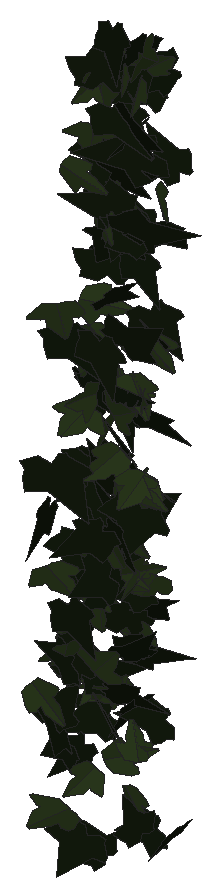
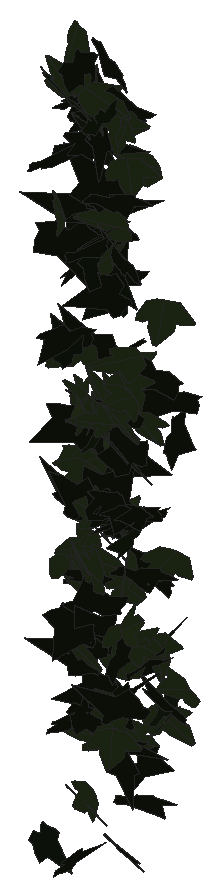
# SketchUp Ruby script. Lengths in inches.
U = 1.inch
M = Sketchup.active_model
def pt(a) = Geom::Point3d.new(a.map { |v| v * U })
def face(e, loops, mat)
  f = e.add_face(loops[0].map { |a| pt(a) })
  loops[1..].each { |l| e.add_face(l.map { |a| pt(a) }).erase! }
  f.material = f.back_material = mat if mat
  f
end
# faces: each face lists its corners as indices into pts; further lists are holes
def faces(e, pts, list, mat = nil) = list.each { |f| face(e, (f[0].is_a?(Array) ? f : [f]).map { |l| l.map { |i| pts[i] } }, mat) }
# xy, xz, yz: faces in a plane at the given z, y or x. An outline is a flat list of corners, or four numbers for a rectangle; further outlines are holes
def ring(l) = l.size == 4 ? [[l[0], l[1]], [l[2], l[1]], [l[2], l[3]], [l[0], l[3]]] : l.each_slice(2).to_a
def flat(e, list, mat, &to3) = list.each { |f| face(e, (f[0].is_a?(Array) ? f : [f]).map { |l| ring(l).map { |u, v| to3.(u, v) } }, mat) }
def xy(e, z, list, mat = nil) = flat(e, list, mat) { |x, y| [x, y, z] }
def xz(e, y, list, mat = nil) = flat(e, list, mat) { |x, z| [x, y, z] }
def yz(e, x, list, mat = nil) = flat(e, list, mat) { |y, z| [x, y, z] }
def lines(e, pts, list) = list.each { |a, b| e.add_line(pt(pts[a]), pt(pts[b])) }
# prism: a flat outline (further loops are holes) pulled along v
def prism(e, loops, v, mat = nil)
  f = face(e, loops, mat); d = Geom::Vector3d.new(v.map { |x| x * U })
  f.pushpull(f.normal.samedirection?(d) ? d.length : -d.length)
end
def box(e, o, s, mat = nil) = prism(e, [[o, [o[0] + s[0], o[1], o[2]], [o[0] + s[0], o[1] + s[1], o[2]], [o[0], o[1] + s[1], o[2]]]], [0, 0, s[2]], mat)
def at(x, y, z, deg = 0) = Geom::Transformation.translation(pt([x, y, z])) * Geom::Transformation.rotation(ORIGIN, Z_AXIS, deg.degrees)
def axes(o, x, y, z) = Geom::Transformation.new([*x, 0, *y, 0, *z, 0, *pt(o).to_a, 1])
def part(name) = M.definitions.add(name)
# library, detail: a bought-in or finely detailed component or shape, given as its bounding box
def library(name, o, s) = part(name).tap { |d| box(d.entities, o, s) }
def detail(e, o, s) = box(e.add_group.entities, o, s)
def put(e, d, t, mat = nil) = e.add_instance(d, t).tap { |i| i.material = mat if mat }
def group(e, t, mat = nil) = e.add_group.tap { |g| g.transformation = t; g.material = mat if mat }.entities
root = M.entities
M.materials.add("1026 AP 7946 SUNNY SIDE UP").color = [254, 231, 186]
M.materials.add("efeu1").color = [18, 25, 13]
M.materials.add("efeu2").color = [43, 57, 29]
c1 = part("ivyleaf_10")
p = [[0,0.5,-0.03],[-0.0625,2.02,-0.43],[-0.19,2.01,-0.46],[-0.54,1.05,-0.29],[-0.52,0.625,-0.18],[-0.83,0.76,-0.28],
  [-1.16,0.64,-0.33],[-1.15,0.33,-0.24],[-0.77,-0.39,0.02],[-0.3,-0.51,0.16],[0.04,-0.48,0.23],[-0.02,2.01,-0.4375],
  [-0.06,2.01,-0.43],[0.04,-0.49,0.23],[0.67,-0.49,0.14],[1.38,0.36,-0.2],[1.375,0.51,-0.24],[0.81,0.65,-0.19],
  [0.62,0.59,-0.15],[0.6,1.09,-0.28],[0.5,1.23,-0.31]]
faces(c1.entities,p,[[0,1,2,3,4,5,6,7,8,9,10],[11,12,0,13,14,15,16,17,18,19,20]],"efeu2")
c2 = part("ivyleaf_9")
p = [[1.54,2.16,1.25],[1.36,2.04,1.19],[-0.21,0.99,0.68],[-0.71,1.11,0.82],[-0.85,0.86,0.67],[-0.8,0.17,0.21],
  [-0.9,-0.01,0.1],[-0.67,-0.16,-0.02],[-0.08,-0.08,-0.05],[-0.03,-0.6,-0.4],[0.65,-0.88,-0.66],[0.83,-0.6,-0.49],
  [1.29,-0.42,-0.43],[1.8125,-0.07,-0.26],[1.21,0.44,0.15]]
faces(c2.entities,p,[[0,1,2,3,4,5,6,7,8,9,10,11,12,13,14]],"efeu1")
put(root,c1,axes([117.14,209.02,253.63],[-0.27587,-0.09025,0.21248],[-0.2515,-0.13497,-0.20129],[0.25018,-0.23519,0.03195]),"1026 AP 7946 SUNNY SIDE UP")
put(root,c2,axes([116.72,209.19,259.3],[-0.09999,0.04613,-0.32791],[0.33476,-0.23752,-0.08061],[-0.37961,-0.22161,0.01529]),"1026 AP 7946 SUNNY SIDE UP")
put(root,c2,axes([116.73,209.31,260.1],[-0.08354,-0.22855,-0.23884],[0.13648,0.21511,-0.23903],[0.49187,-0.09851,0.02576]),"1026 AP 7946 SUNNY SIDE UP")
put(root,c2,axes([117.36,209.79,258.8125],[-0.01614,-0.03063,-0.29387],[0.02416,-0.28492,0.0293],[-0.4502,-0.01419,0.01211]),"1026 AP 7946 SUNNY SIDE UP")
put(root,c2,axes([116.63,209.875,257.04],[-0.13329,-0.07492,-0.27678],[0.42285,0.05093,-0.10191],[0.11393,-0.27667,0.0544]),"1026 AP 7946 SUNNY SIDE UP")
put(root,c2,axes([117.24,210.14,257.74],[-0.16853,-0.15358,0.22708],[-0.17197,-0.19285,-0.19357],[0.38707,-0.15254,0.01287]),"1026 AP 7946 SUNNY SIDE UP")
put(root,c2,axes([116.16,210.13,254.47],[-0.02015,-0.19103,0.2175],[0.01022,-0.21257,-0.19797],[0.44885,-0.00374,0.01427]),"1026 AP 7946 SUNNY SIDE UP")
put(root,c2,axes([116.83,210.07,252.57],[-0.34327,-0.1662,0.00271],[0.01829,-0.02116,-0.28171],[0.26076,-0.21731,0.02333]),"1026 AP 7946 SUNNY SIDE UP")
put(root,c1,axes([115.79,210.04,255.05],[0.24848,0.01045,0.24141],[0.3686,-0.01472,-0.16231],[0.01003,0.2822,-0.01575]),"1026 AP 7946 SUNNY SIDE UP")
put(root,c1,axes([116.86,210.15,253.78],[0.15228,0.13186,-0.22572],[-0.17084,-0.19175,-0.16891],[-0.36512,0.14472,-0.01511]),"1026 AP 7946 SUNNY SIDE UP")
put(root,c2,axes([116.27,210.23,254.125],[0.13204,-0.16753,-0.18657],[0.14401,-0.15539,0.19193],[-0.35903,-0.12394,0.00837]),"1026 AP 7946 SUNNY SIDE UP")
put(root,c1,axes([116.77,210.31,261.03],[-0.00319,-0.02129,-0.30481],[-0.14173,-0.28172,0.01989],[-0.44418,0.09004,-0.00415]),"1026 AP 7946 SUNNY SIDE UP")
put(root,c1,axes([116.09,210.06,257.49],[-0.28402,-0.16723,-0.15757],[0.21516,0.07393,-0.25088],[0.2828,-0.2242,0.03263]),"1026 AP 7946 SUNNY SIDE UP")
put(root,c2,axes([116.29,210.31,255.66],[0.07807,-0.27122,-0.04217],[0.04896,-0.03419,0.28275],[-0.42815,-0.05336,0.02465]),"1026 AP 7946 SUNNY SIDE UP")
put(root,c1,axes([116.8,210.42,258.17],[-0.04534,-0.03091,-0.3116],[-0.03095,-0.30283,0.03206],[-0.4768,0.0226,0.02755]),"1026 AP 7946 SUNNY SIDE UP")
put(root,c2,axes([116.07,210.14,254.59],[-0.25331,0.18158,0.13881],[0.15811,-0.08925,0.24913],[0.31737,0.18939,-0.01332]),"1026 AP 7946 SUNNY SIDE UP")
put(root,c1,axes([116.19,210.3125,255.9],[-0.12614,-0.28371,-0.00245],[0.01409,-0.00173,-0.30361],[0.44589,-0.08021,0.0089]),"1026 AP 7946 SUNNY SIDE UP")
put(root,c1,axes([116.03,210.33,262.46],[-0.31797,-0.22697,-0.0564],[0.08029,0.02594,-0.3123],[0.35776,-0.20755,0.01996]),"1026 AP 7946 SUNNY SIDE UP")
put(root,c2,axes([117.1875,210.2,257.38],[-0.14759,0.20647,0.2165],[-0.19574,0.17077,-0.23041],[-0.41842,-0.15272,0.03142]),"1026 AP 7946 SUNNY SIDE UP")
put(root,c1,axes([116.25,210.42,265.21],[-0.10638,0.00375,-0.27373],[0.38081,-0.11203,-0.0658],[-0.17206,-0.25028,0.0236]),"1026 AP 7946 SUNNY SIDE UP")
put(root,c1,axes([117.05,210.57,259.84],[0.17054,0.13451,-0.26301],[-0.20999,-0.2193,-0.17823],[-0.40343,0.17101,-0.01842]),"1026 AP 7946 SUNNY SIDE UP")
put(root,c1,axes([117.24,210.38,257.99],[-0.30246,0.10376,-0.17073],[-0.20535,0.10594,0.22431],[0.22987,0.23117,-0.02426]),"1026 AP 7946 SUNNY SIDE UP")
put(root,c2,axes([116.91,210.61,258.34],[0.00271,-0.03807,-0.2683],[0.41353,0.00019,0.00177],[-0.0001,-0.26023,0.0377]),"1026 AP 7946 SUNNY SIDE UP")
put(root,c2,axes([116.68,210.74,254.68],[0.261,-0.11787,-0.21168],[0.29417,-0.08735,0.20748],[-0.227,-0.24874,0.02549]),"1026 AP 7946 SUNNY SIDE UP")
put(root,c2,axes([116.32,210.55,255.4],[-0.23653,-0.2084,0.13365],[0.09868,0.11588,0.265],[-0.3742,0.16229,-0.0146]),"1026 AP 7946 SUNNY SIDE UP")
put(root,c2,axes([116.18,210.79,253.8],[-0.0096,-0.02293,-0.27412],[0.14416,-0.25002,0.01858],[-0.39421,-0.09087,0.01347]),"1026 AP 7946 SUNNY SIDE UP")
put(root,c1,axes([116.29,210.67,260.4],[0.38275,0.03573,-0.11445],[-0.16622,-0.04246,-0.25247],[-0.07846,0.26427,-0.02348]),"1026 AP 7946 SUNNY SIDE UP")
put(root,c1,axes([117.47,210.75,259.4375],[0.27152,0.16457,-0.16021],[-0.15244,-0.1243,-0.24566],[-0.32286,0.19709,-0.01875]),"1026 AP 7946 SUNNY SIDE UP")
put(root,c1,axes([116.96,210.75,260.53],[-0.26045,0.08066,0.21171],[0.31167,-0.0575,0.18791],[0.15133,0.25724,-0.02266]),"1026 AP 7946 SUNNY SIDE UP")
put(root,c2,axes([117.17,210.88,266.18],[0.08158,-0.12578,0.31658],[0.21236,-0.27694,-0.14156],[0.47811,0.14447,0.00886]),"1026 AP 7946 SUNNY SIDE UP")
put(root,c1,axes([116.58,210.71,255.47],[-0.40476,-0.00336,0.14424],[0.21931,0.02082,0.26478],[-0.02028,0.2923,-0.01548]),"1026 AP 7946 SUNNY SIDE UP")
put(root,c1,axes([116.39,210.7,256.99],[0.21635,-0.0614,-0.24398],[0.37271,-0.03225,0.15051],[-0.09314,-0.27169,0.03557]),"1026 AP 7946 SUNNY SIDE UP")
put(root,c2,axes([117.4,210.86,258.79],[-0.3702,-0.16495,-0.08726],[0.1318,0.02575,-0.29479],[0.25933,-0.24856,0.02526]),"1026 AP 7946 SUNNY SIDE UP")
put(root,c1,axes([116.52,210.89,264.13],[-0.1225,0.01738,-0.26626],[0.19678,-0.23389,-0.05641],[-0.3568,-0.13496,0.0603]),"1026 AP 7946 SUNNY SIDE UP")
put(root,c2,axes([116.5,210.87,261.71],[0.02181,-0.30711,-0.02043],[-0.00582,0.01793,-0.31658],[0.4837,0.01407,-0.00289]),"1026 AP 7946 SUNNY SIDE UP")
put(root,c2,axes([116.77,210.91,260.02],[0.30694,-0.10214,-0.19229],[0.27723,-0.06274,0.22566],[-0.18585,-0.26228,0.01905]),"1026 AP 7946 SUNNY SIDE UP")
put(root,c1,axes([117.34,210.98,257.48],[0.0648,-0.121,0.2679],[0.09045,-0.2546,-0.13257],[0.44284,0.06971,-0.01213]),"1026 AP 7946 SUNNY SIDE UP")
put(root,c1,axes([117.27,210.76,259.3],[-0.23336,-0.04401,-0.22178],[0.34511,-0.02765,-0.15039],[0.00279,-0.2598,0.05199]),"1026 AP 7946 SUNNY SIDE UP")
put(root,c1,axes([116.69,210.84,257.44],[-0.07207,-0.03243,-0.31994],[0.45525,-0.12148,-0.03168],[-0.1831,-0.28927,0.04716]),"1026 AP 7946 SUNNY SIDE UP")
put(root,c1,axes([117.07,210.6,253.9375],[-0.05933,-0.07568,0.29038],[0.15754,0.26405,0.08827],[-0.43172,0.10676,-0.00769]),"1026 AP 7946 SUNNY SIDE UP")
put(root,c1,axes([116.05,210.98,256.24],[-0.06155,-0.15669,0.23426],[-0.02642,-0.22878,-0.16608],[0.43457,-0.0361,0.02308]),"1026 AP 7946 SUNNY SIDE UP")
put(root,c2,axes([116.74,210.68,251.9375],[-0.30893,0.02715,-0.15592],[-0.22741,0.05151,0.20303],[0.08283,0.2427,-0.02414]),"1026 AP 7946 SUNNY SIDE UP")
put(root,c2,axes([116.11,210.94,257.62],[-0.29799,-0.20196,-0.05598],[0.07843,0.02598,-0.28454],[0.31888,-0.19511,0.01767]),"1026 AP 7946 SUNNY SIDE UP")
put(root,c2,axes([116.85,210.97,264.39],[-0.14411,-0.0081,0.27555],[-0.39704,-0.09112,-0.09249],[0.1395,-0.2677,0.0214]),"1026 AP 7946 SUNNY SIDE UP")
put(root,c2,axes([116.89,210.82,263.98],[0.217,0.11977,-0.21034],[-0.21849,-0.15131,-0.18845],[-0.30246,0.19523,-0.01477]),"1026 AP 7946 SUNNY SIDE UP")
put(root,c1,axes([116.47,210.68,257.6],[0.04955,-0.20284,-0.2458],[0.00387,0.23881,-0.20842],[0.49103,0.01859,0.02645]),"1026 AP 7946 SUNNY SIDE UP")
put(root,c1,axes([117.36,210.78,254.08],[0.11252,0.24311,-0.05161],[-0.00083,0.05372,0.2609],[0.39074,-0.06989,0.01542]),"1026 AP 7946 SUNNY SIDE UP")
put(root,c2,axes([117.49,210.74,252.62],[-0.31966,0.05052,-0.15601],[-0.21798,0.06666,0.21461],[0.12535,0.24475,-0.02465]),"1026 AP 7946 SUNNY SIDE UP")
put(root,c2,axes([116.36,211.02,255.11],[-0.01709,-0.24334,-0.05394],[0.01895,-0.05148,0.25021],[-0.39047,0.00815,0.01451]),"1026 AP 7946 SUNNY SIDE UP")
put(root,c1,axes([117.32,210.69,257.58],[0.06555,-0.0387,0.2792],[0.07133,0.27155,0.03432],[-0.42487,0.03962,0.04884]),"1026 AP 7946 SUNNY SIDE UP")
put(root,c2,axes([117.28,210.97,264.02],[-0.26888,-0.23193,-0.05288],[-0.0678,-0.03024,0.29619],[-0.36685,0.17558,-0.01599]),"1026 AP 7946 SUNNY SIDE UP")
put(root,c1,axes([117.21,210.9,259.13],[-0.40527,0.00162,-0.14134],[0.21448,-0.0288,-0.26447],[-0.02351,-0.29056,0.02371]),"1026 AP 7946 SUNNY SIDE UP")
put(root,c2,axes([115.78,210.91,261.62],[-0.12101,-0.10607,-0.28417],[0.32433,0.18399,-0.13139],[0.33156,-0.21869,0.02481]),"1026 AP 7946 SUNNY SIDE UP")
put(root,c2,axes([117.31,211.15,265.6],[-0.0828,-0.1669,-0.29798],[-0.16667,-0.26832,0.17839],[-0.49658,0.11788,-0.01019]),"1026 AP 7946 SUNNY SIDE UP")
put(root,c2,axes([117.32,211.07,257.12],[-0.28561,-0.02784,0.20371],[-0.29001,-0.07962,-0.1864],[0.121,-0.25655,0.03408]),"1026 AP 7946 SUNNY SIDE UP")
put(root,c2,axes([117.12,210.84,264.12],[0.16148,0.02947,0.30579],[0.46875,-0.01255,-0.1051],[0.00358,0.31368,-0.03108]),"1026 AP 7946 SUNNY SIDE UP")
put(root,c2,axes([116.75,210.73,262.76],[0.17926,0.19627,0.1556],[0.13282,0.12418,-0.23292],[-0.36493,0.14161,-0.00835]),"1026 AP 7946 SUNNY SIDE UP")
put(root,c2,axes([116.91,210.88,258.29],[0.10197,-0.06084,0.24936],[-0.19499,0.20959,0.0896],[-0.34118,-0.13797,0.02332]),"1026 AP 7946 SUNNY SIDE UP")
put(root,c2,axes([116.99,210.94,255.78],[0.29265,0.18795,0.04604],[-0.07072,-0.01668,0.27162],[0.29502,-0.19043,0.01944]),"1026 AP 7946 SUNNY SIDE UP")
put(root,c2,axes([116.43,211.15,258.55],[-0.09496,-0.27369,0.06435],[-0.00622,-0.06464,-0.28893],[0.44192,-0.05972,0.00976]),"1026 AP 7946 SUNNY SIDE UP")
put(root,c2,axes([116.73,210.97,266.29],[-0.00405,-0.21427,-0.19925],[0.14728,0.18112,-0.20825],[0.42796,-0.06436,0.06978]),"1026 AP 7946 SUNNY SIDE UP")
put(root,c2,axes([115.81,211,258.79],[0.0821,-0.25655,-0.12069],[-0.01715,0.11573,-0.26878],[0.44219,0.05212,0.01198]),"1026 AP 7946 SUNNY SIDE UP")
put(root,c1,axes([117.5,211.05,257.37],[-0.29654,-0.17294,0.10028],[-0.09212,-0.08119,-0.26336],[0.29894,-0.19657,0.01831]),"1026 AP 7946 SUNNY SIDE UP")
put(root,c2,axes([116.74,210.92,255.01],[0.33277,0.02752,0.14496],[0.22312,-0.00627,-0.21888],[-0.03055,0.25398,-0.01961]),"1026 AP 7946 SUNNY SIDE UP")
put(root,c2,axes([116.77,210.91,265.5625],[-0.02846,0.26602,0.04801],[0.00563,-0.04495,0.27442],[0.42421,0.01845,-0.00042]),"1026 AP 7946 SUNNY SIDE UP")
put(root,c1,axes([117.15,211.18,266.83],[-0.04749,0.16285,-0.22179],[-0.02259,-0.21821,-0.16852],[-0.42502,-0.0066,0.03374]),"1026 AP 7946 SUNNY SIDE UP")
put(root,c2,axes([116.36,211.19,254.27],[-0.33757,-0.08274,0.12658],[-0.16634,-0.067,-0.23637],[0.16393,-0.23836,0.02083]),"1026 AP 7946 SUNNY SIDE UP")
put(root,c2,axes([116.6875,211.07,258.88],[0.25426,-0.09069,0.23702],[-0.27211,0.15573,0.18903],[-0.27885,-0.23466,0.03166]),"1026 AP 7946 SUNNY SIDE UP")
put(root,c1,axes([117.01,211.11,253.01],[-0.26568,0.13695,-0.15313],[0.15139,-0.11695,-0.22327],[-0.28045,-0.19287,0.02454]),"1026 AP 7946 SUNNY SIDE UP")
put(root,c2,axes([116.6,210.95,263.11],[-0.35359,-0.04469,0.18088],[0.25965,0.06556,0.23511],[-0.11815,0.27782,-0.02463]),"1026 AP 7946 SUNNY SIDE UP")
put(root,c1,axes([116.51,211.02,254.78],[-0.13402,-0.19637,0.11857],[0.06264,0.10934,0.22108],[-0.35328,0.09388,-0.00578]),"1026 AP 7946 SUNNY SIDE UP")
put(root,c1,axes([116.47,211.21,260.07],[0.12227,-0.24765,0.14468],[0.05241,-0.13813,-0.26807],[0.44568,0.08418,-0.00817]),"1026 AP 7946 SUNNY SIDE UP")
put(root,c2,axes([116.67,211.29,264.05],[-0.11587,-0.26551,0.1163],[-0.0224,-0.11458,-0.28408],[0.45403,-0.07341,0.01566]),"1026 AP 7946 SUNNY SIDE UP")
put(root,c2,axes([117.24,211.1,258.54],[-0.12816,0.12282,0.25983],[0.27036,-0.18474,0.14925],[0.34729,0.18914,-0.02031]),"1026 AP 7946 SUNNY SIDE UP")
put(root,c1,axes([116.22,211.18,261.36],[-0.24045,-0.20902,0.10749],[-0.0691,-0.09818,-0.26652],[0.36164,-0.15774,0.02055]),"1026 AP 7946 SUNNY SIDE UP")
put(root,c2,axes([116.8125,211.18,261.66],[-0.13387,0.00908,0.28919],[0.34326,-0.18233,0.07323],[0.27773,0.22973,0.04888]),"1026 AP 7946 SUNNY SIDE UP")
put(root,c2,axes([116.19,211.16,260.52],[0.11636,-0.00611,0.28803],[0.38286,-0.14093,-0.07038],[0.21641,0.2526,-0.03036]),"1026 AP 7946 SUNNY SIDE UP")
put(root,c2,axes([116.55,211.1875,264.93],[0.42438,-0.00112,-0.13553],[0.20312,0.05913,0.27285],[0.03919,-0.29437,0.05353]),"1026 AP 7946 SUNNY SIDE UP")
put(root,c1,axes([117.01,211.28,260.79],[-0.10053,0.02737,0.25893],[0.30469,-0.16097,0.06794],[0.25498,0.20315,0.0209]),"1026 AP 7946 SUNNY SIDE UP")
put(root,c1,axes([116.27,211.125,256.43],[-0.20367,-0.25414,-0.05329],[0.06117,0.0365,-0.29307],[0.40274,-0.13407,0.01756]),"1026 AP 7946 SUNNY SIDE UP")
put(root,c1,axes([117.38,210.96,267.6],[-0.02223,-0.20533,-0.27909],[0.03865,0.26865,-0.21042],[0.53164,-0.02812,0.00363]),"1026 AP 7946 SUNNY SIDE UP")
put(root,c2,axes([117.06,211.21,254.77],[-0.11574,0.16292,-0.1979],[0.10898,-0.18031,-0.18507],[-0.38193,-0.10082,0.00716]),"1026 AP 7946 SUNNY SIDE UP")
put(root,c1,axes([115.97,211.36,256.73],[0.02947,-0.0502,0.28789],[0.14872,-0.26326,-0.05673],[0.42141,0.09642,-0.00011]),"1026 AP 7946 SUNNY SIDE UP")
put(root,c2,axes([116.45,211.28,267.6],[-0.23664,-0.0152,-0.26817],[0.40793,-0.03802,-0.1525],[-0.03994,-0.2982,0.03134]),"1026 AP 7946 SUNNY SIDE UP")
put(root,c1,axes([116.04,211.34,266.45],[0.06247,0.10697,-0.25251],[-0.13802,-0.2295,-0.1189],[-0.39814,0.09634,0.00159]),"1026 AP 7946 SUNNY SIDE UP")
put(root,c1,axes([116.75,211.34,260.62],[-0.01889,0.10097,-0.26525],[0.04266,-0.25662,-0.10624],[-0.43361,-0.02964,0.0011]),"1026 AP 7946 SUNNY SIDE UP")
put(root,c2,axes([117.03,211.22,263.42],[0.0933,-0.25983,-0.08698],[-0.03259,0.08035,-0.27409],[0.42764,0.06281,-0.00191]),"1026 AP 7946 SUNNY SIDE UP")
put(root,c1,axes([116.72,211.3125,267.06],[-0.05724,0.17996,-0.20826],[0.01619,-0.20393,-0.18918],[-0.42647,-0.03189,0.02077]),"1026 AP 7946 SUNNY SIDE UP")
put(root,c1,axes([116.22,211.31,260.91],[-0.24227,0.05585,0.25508],[0.34021,-0.12184,0.16652],[0.20775,0.26466,0.02477]),"1026 AP 7946 SUNNY SIDE UP")
put(root,c1,axes([116.08,211.22,265.6],[-0.29603,-0.19308,0.01999],[-0.00126,-0.02778,-0.27731],[0.30531,-0.18733,0.01824]),"1026 AP 7946 SUNNY SIDE UP")
put(root,c2,axes([116.49,211.32,258.82],[0.20086,-0.16333,0.13707],[0.11484,-0.11277,-0.21403],[0.31169,0.1468,-0.00948]),"1026 AP 7946 SUNNY SIDE UP")
put(root,c2,axes([116.5,211.41,260.33],[0.08468,-0.27118,0.13002],[0.02797,-0.12667,-0.28549],[0.47052,0.05633,-0.00642]),"1026 AP 7946 SUNNY SIDE UP")
put(root,c1,axes([116.3,211.2,264.36],[0.06258,0.04164,0.30206],[0.44577,0.07939,-0.05083],[-0.13341,0.28481,-0.02816]),"1026 AP 7946 SUNNY SIDE UP")
put(root,c2,axes([116.92,211.16,255.74],[0.19046,0.00349,0.26278],[0.40072,-0.01384,-0.12456],[0.0173,0.28202,-0.00771]),"1026 AP 7946 SUNNY SIDE UP")
put(root,c2,axes([117.39,211.46,254.43],[-0.0154,-0.20691,-0.15423],[-0.01321,-0.1483,0.21253],[-0.40028,0.01286,-0.00108]),"1026 AP 7946 SUNNY SIDE UP")
put(root,c2,axes([116.86,211.16,256.24],[-0.18915,-0.0895,0.24613],[0.31126,0.13479,0.15516],[-0.25428,0.23158,0.00683]),"1026 AP 7946 SUNNY SIDE UP")
put(root,c2,axes([115.88,211.36,258.49],[0.19413,-0.20889,0.02871],[0.00681,-0.03115,-0.24985],[0.33156,0.12295,-0.01168]),"1026 AP 7946 SUNNY SIDE UP")
put(root,c1,axes([116.84,211.33,260.86],[0.34831,0.0067,0.17281],[0.26291,-0.03295,-0.22636],[0.02294,0.27588,-0.0296]),"1026 AP 7946 SUNNY SIDE UP")
put(root,c2,axes([115.88,211.34,259.05],[-0.10946,-0.23305,-0.14736],[0.09111,0.13029,-0.24928],[0.41909,-0.08919,0.0157]),"1026 AP 7946 SUNNY SIDE UP")
put(root,c2,axes([116.58,211.36,263.67],[-0.13592,0.21992,-0.20504],[0.06796,-0.19707,-0.24329],[-0.46275,-0.09353,0.0245]),"1026 AP 7946 SUNNY SIDE UP")
put(root,c2,axes([116.3,211.19,266.65],[-0.43277,0.04838,0.09746],[0.15314,0.01175,0.28661],[0.06584,0.29071,-0.02605]),"1026 AP 7946 SUNNY SIDE UP")
put(root,c2,axes([116.84,211.43,258.79],[0.0792,-0.04916,0.29145],[0.25687,-0.23166,-0.07272],[0.37185,0.1705,-0.01185]),"1026 AP 7946 SUNNY SIDE UP")
put(root,c1,axes([116.21,211.41,254.77],[0.28061,0.12031,-0.16563],[-0.18772,-0.11052,-0.22142],[-0.25496,0.21378,-0.01927]),"1026 AP 7946 SUNNY SIDE UP")
put(root,c1,axes([117.15,211.3,261.82],[-0.39781,-0.06637,-0.15573],[0.23967,0.01059,-0.2682],[0.09833,-0.29433,0.02366]),"1026 AP 7946 SUNNY SIDE UP")
put(root,c2,axes([117.13,211.54,266.64],[-0.22355,-0.12099,0.18585],[-0.15911,-0.1548,-0.1893],[0.30325,-0.17042,0.03768]),"1026 AP 7946 SUNNY SIDE UP")
put(root,c2,axes([115.99,211.3,255],[0.04969,0.01956,0.2731],[0.40361,-0.0712,-0.02654],[0.10795,0.25719,-0.02649]),"1026 AP 7946 SUNNY SIDE UP")
put(root,c2,axes([116.73,211.31,256.82],[-0.31259,-0.08877,0.19701],[0.29206,0.05208,0.22353],[-0.15838,0.27124,0.02337]),"1026 AP 7946 SUNNY SIDE UP")
put(root,c1,axes([116.1875,211.35,266.46],[-0.3854,0.10799,0.03906],[-0.06787,-0.00578,-0.27498],[-0.16633,-0.24786,0.02171]),"1026 AP 7946 SUNNY SIDE UP")
put(root,c1,axes([116.76,211.24,258.65],[0.03971,-0.19738,0.22235],[-0.05142,0.21451,0.20622],[-0.45832,-0.04117,-0.00387]),"1026 AP 7946 SUNNY SIDE UP")
put(root,c1,axes([117.16,211.32,256.04],[0.14654,-0.07621,-0.24039],[-0.29906,0.13465,-0.123],[0.243,0.21167,-0.00641]),"1026 AP 7946 SUNNY SIDE UP")
put(root,c2,axes([116.2,211.54,265.09],[-0.30008,-0.21474,-0.04411],[0.06675,0.01779,-0.29516],[0.33739,-0.19451,0.01916]),"1026 AP 7946 SUNNY SIDE UP")
put(root,c2,axes([116,211.62,256.33],[-0.0074,-0.01991,-0.31822],[0.31166,-0.23733,0.01126],[-0.3736,-0.19759,0.0157]),"1026 AP 7946 SUNNY SIDE UP")
put(root,c2,axes([117.06,211.52,261.8],[0.30512,-0.07207,-0.14598],[0.22177,-0.02373,0.21188],[-0.1141,-0.23886,0.02146]),"1026 AP 7946 SUNNY SIDE UP")
put(root,c2,axes([117.05,211.32,260.31],[0.3855,0.03333,0.07497],[0.11685,-0.00935,-0.25424],[-0.04601,0.25552,-0.01756]),"1026 AP 7946 SUNNY SIDE UP")
put(root,c2,axes([116.57,211.35,266.15],[0.25026,-0.05964,-0.22078],[-0.33467,0.03438,-0.17277],[0.09994,0.26445,-0.02568]),"1026 AP 7946 SUNNY SIDE UP")
put(root,c2,axes([117.17,211.43,264.02],[0.22171,0.18711,-0.23897],[-0.18755,-0.20102,-0.24181],[-0.43086,0.18378,-0.01771]),"1026 AP 7946 SUNNY SIDE UP")
put(root,c2,axes([116.9375,211.5625,267.45],[-0.09162,0.12527,-0.24084],[0.10918,-0.22456,-0.14267],[-0.40353,-0.0892,0.01608]),"1026 AP 7946 SUNNY SIDE UP")
put(root,c2,axes([116.01,211.43,259.16],[-0.05762,-0.11169,-0.27617],[0.27867,0.20466,-0.11187],[0.36059,-0.17601,0.04232]),"1026 AP 7946 SUNNY SIDE UP")
put(root,c1,axes([116.59,211.56,266.71],[0.24301,-0.26495,0.05798],[0.0233,-0.05816,-0.31589],[0.42576,0.1544,-0.01581]),"1026 AP 7946 SUNNY SIDE UP")
put(root,c2,axes([116.15,211.49,260.29],[-0.3219,0.13331,-0.03165],[0.0234,-0.03462,-0.25097],[-0.2141,-0.20421,0.02015]),"1026 AP 7946 SUNNY SIDE UP")
put(root,c1,axes([116.51,211.59,267.01],[-0.20545,-0.09956,0.22945],[-0.22848,-0.17199,-0.1676],[0.30916,-0.19327,0.02862]),"1026 AP 7946 SUNNY SIDE UP")
put(root,c1,axes([116.21,211.67,263.92],[-0.08572,0.03712,0.2731],[0.11148,-0.25865,0.05086],[0.40553,0.07895,0.04375]),"1026 AP 7946 SUNNY SIDE UP")
put(root,c2,axes([116.28,211.68,266.62],[0.04816,-0.19208,0.2248],[0.10553,-0.20994,-0.20031],[0.44609,0.0704,0.02312]),"1026 AP 7946 SUNNY SIDE UP")
put(root,c2,axes([116.07,211.42,254.2],[0.20366,-0.01832,-0.24217],[-0.37057,-0.01198,-0.13294],[-0.00264,0.26803,-0.02092]),"1026 AP 7946 SUNNY SIDE UP")
put(root,c1,axes([116.98,211.32,260.49],[0.09252,-0.09172,0.23981],[-0.14147,0.21595,0.1121],[-0.36792,-0.1061,0.0172]),"1026 AP 7946 SUNNY SIDE UP")
put(root,c1,axes([116.23,211.47,260.91],[0.23398,-0.1176,-0.19493],[-0.26133,0.09172,-0.19353],[0.23194,0.22199,-0.02141]),"1026 AP 7946 SUNNY SIDE UP")
put(root,c1,axes([116.3125,211.36,260.59],[-0.01591,0.02443,0.28266],[0.29097,0.2038,-0.01048],[-0.32056,0.18378,-0.02354]),"1026 AP 7946 SUNNY SIDE UP")
put(root,c1,axes([116.41,211.62,257.69],[0.00478,-0.00734,0.32278],[0.45995,-0.11253,-0.0063],[0.17709,0.29247,0.00764]),"1026 AP 7946 SUNNY SIDE UP")
put(root,c1,axes([117.17,211.68,264.49],[-0.06723,0.06696,-0.27835],[0.1628,-0.25033,-0.08214],[-0.40692,-0.11122,0.01312]),"1026 AP 7946 SUNNY SIDE UP")
put(root,c2,axes([117.65,211.54,265.22],[-0.24231,-0.21194,0.07714],[0.04825,0.07156,0.26984],[-0.35078,0.15625,-0.01617]),"1026 AP 7946 SUNNY SIDE UP")
put(root,c2,axes([115.68,211.65,260.22],[0.41605,-0.07421,-0.08571],[0.14107,0.01634,0.28044],[-0.10324,-0.27676,0.0378]),"1026 AP 7946 SUNNY SIDE UP")
put(root,c1,axes([117.02,211.59,266.96],[-0.31863,-0.06337,0.15362],[0.23283,0.02593,0.21826],[-0.10472,0.25047,0.01785]),"1026 AP 7946 SUNNY SIDE UP")
put(root,c2,axes([116.97,211.78,252.01],[0.04098,-0.20226,-0.17119],[0.06651,-0.16038,0.20845],[-0.40503,-0.0468,0.01691]),"1026 AP 7946 SUNNY SIDE UP")
put(root,c1,axes([115.8,211.62,261.38],[-0.27149,0.03774,-0.17508],[0.23402,-0.09272,-0.17731],[-0.14262,-0.22398,0.04233]),"1026 AP 7946 SUNNY SIDE UP")
put(root,c2,axes([117.02,211.42,256.51],[0.21073,0.21561,0.06583],[0.07226,0.04511,-0.26082],[-0.34559,0.1409,-0.01439]),"1026 AP 7946 SUNNY SIDE UP")
put(root,c1,axes([116.59,211.75,257.85],[0.00697,-0.0858,-0.25881],[0.20652,-0.2171,0.07765],[-0.36193,-0.12553,0.03932]),"1026 AP 7946 SUNNY SIDE UP")
put(root,c2,axes([116.76,211.5625,263.76],[-0.30957,-0.17799,0.09078],[0.08272,0.07437,0.27317],[-0.30187,0.20291,-0.01824]),"1026 AP 7946 SUNNY SIDE UP")
put(root,c2,axes([117.59,211.65,252.28],[-0.16963,0.16807,-0.16434],[0.10398,-0.14741,-0.2057],[-0.35029,-0.12514,0.01852]),"1026 AP 7946 SUNNY SIDE UP")
put(root,c1,axes([116.13,211.6,254.67],[-0.30877,-0.19168,-0.02344],[0.04552,0.00128,-0.28199],[0.29988,-0.19755,0.01867]),"1026 AP 7946 SUNNY SIDE UP")
put(root,c1,axes([115.82,211.46,262.0625],[-0.06588,-0.09457,-0.28903],[0.36681,0.16308,-0.09174],[0.28536,-0.23146,0.0512]),"1026 AP 7946 SUNNY SIDE UP")
put(root,c2,axes([116.125,211.48,263.24],[0.30575,0.09001,0.14367],[0.22047,0.02443,-0.2183],[-0.13842,0.23774,-0.03035]),"1026 AP 7946 SUNNY SIDE UP")
put(root,c2,axes([115.83,211.6,263.85],[-0.15463,0.15902,0.19634],[0.15139,-0.16346,0.19163],[0.35855,0.1376,0.00376]),"1026 AP 7946 SUNNY SIDE UP")
put(root,c2,axes([117.38,211.66,267.02],[-0.43004,0.13997,-0.06063],[0.06128,-0.05415,-0.31532],[-0.23125,-0.27463,0.02919]),"1026 AP 7946 SUNNY SIDE UP")
put(root,c2,axes([117.0625,211.58,262.2],[-0.01967,-0.20215,-0.2179],[0.01866,0.21003,-0.20742],[0.45837,-0.01722,-0.00091]),"1026 AP 7946 SUNNY SIDE UP")
